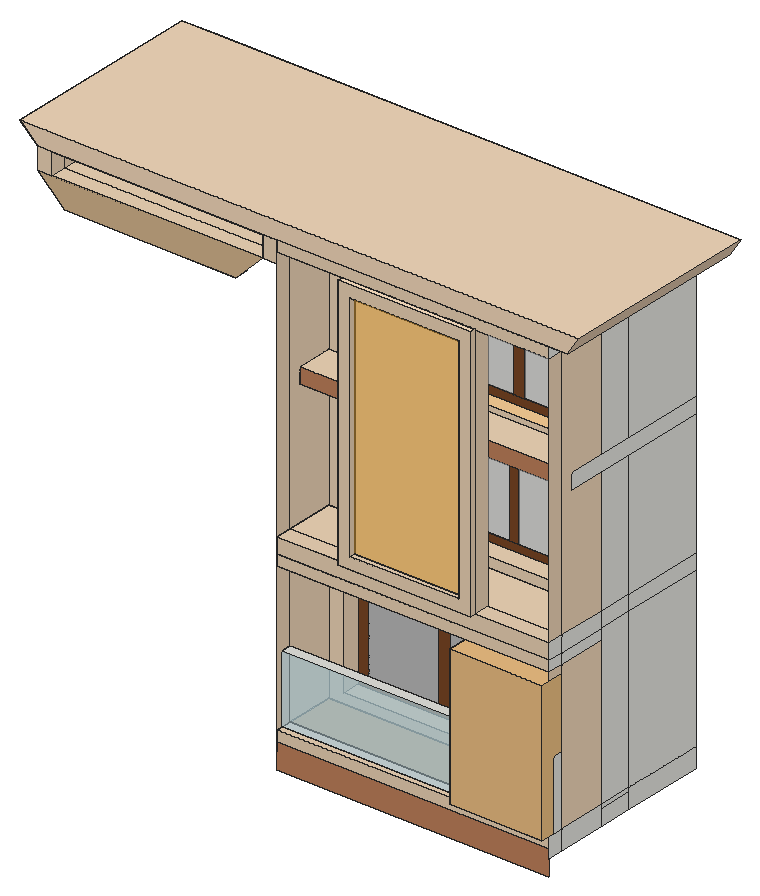
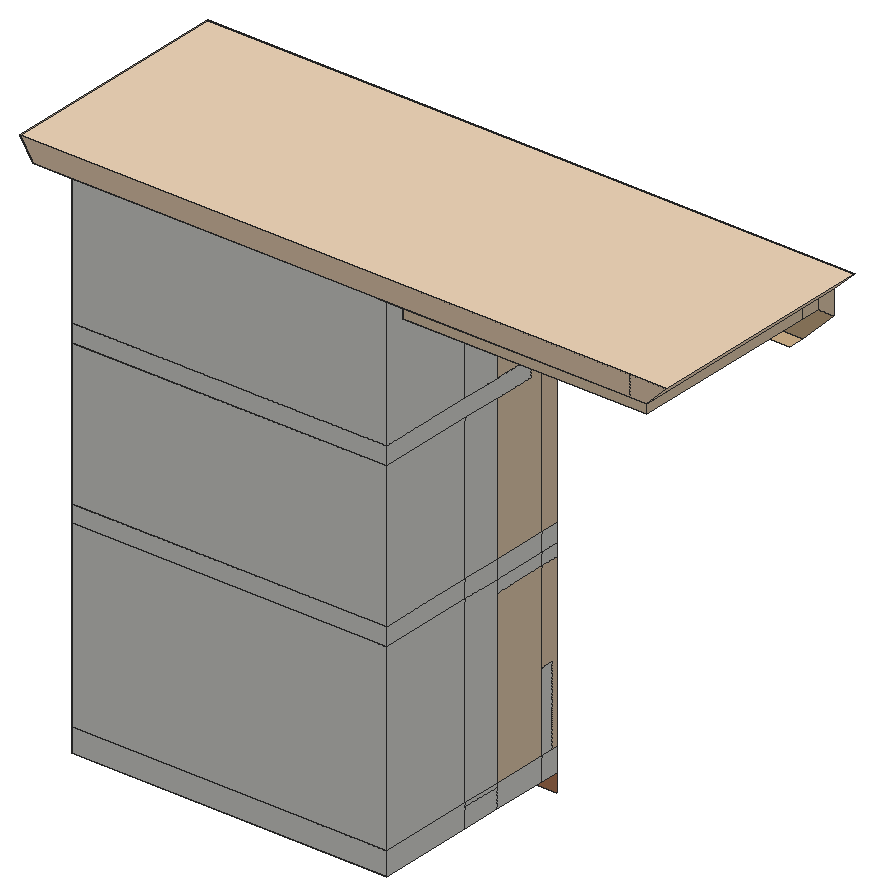
# SketchUp Ruby script. Lengths in inches.
U = 1.inch
M = Sketchup.active_model
def pt(a) = Geom::Point3d.new(a.map { |v| v * U })
def face(e, loops, mat)
  f = e.add_face(loops[0].map { |a| pt(a) })
  loops[1..].each { |l| e.add_face(l.map { |a| pt(a) }).erase! }
  f.material = f.back_material = mat if mat
  f
end
# faces: each face lists its corners as indices into pts; further lists are holes
def faces(e, pts, list, mat = nil) = list.each { |f| face(e, (f[0].is_a?(Array) ? f : [f]).map { |l| l.map { |i| pts[i] } }, mat) }
# xy, xz, yz: faces in a plane at the given z, y or x. An outline is a flat list of corners, or four numbers for a rectangle; further outlines are holes
def ring(l) = l.size == 4 ? [[l[0], l[1]], [l[2], l[1]], [l[2], l[3]], [l[0], l[3]]] : l.each_slice(2).to_a
def flat(e, list, mat, &to3) = list.each { |f| face(e, (f[0].is_a?(Array) ? f : [f]).map { |l| ring(l).map { |u, v| to3.(u, v) } }, mat) }
def xy(e, z, list, mat = nil) = flat(e, list, mat) { |x, y| [x, y, z] }
def xz(e, y, list, mat = nil) = flat(e, list, mat) { |x, z| [x, y, z] }
def yz(e, x, list, mat = nil) = flat(e, list, mat) { |y, z| [x, y, z] }
def lines(e, pts, list) = list.each { |a, b| e.add_line(pt(pts[a]), pt(pts[b])) }
# prism: a flat outline (further loops are holes) pulled along v
def prism(e, loops, v, mat = nil)
  f = face(e, loops, mat); d = Geom::Vector3d.new(v.map { |x| x * U })
  f.pushpull(f.normal.samedirection?(d) ? d.length : -d.length)
end
def box(e, o, s, mat = nil) = prism(e, [[o, [o[0] + s[0], o[1], o[2]], [o[0] + s[0], o[1] + s[1], o[2]], [o[0], o[1] + s[1], o[2]]]], [0, 0, s[2]], mat)
def at(x, y, z, deg = 0) = Geom::Transformation.translation(pt([x, y, z])) * Geom::Transformation.rotation(ORIGIN, Z_AXIS, deg.degrees)
def axes(o, x, y, z) = Geom::Transformation.new([*x, 0, *y, 0, *z, 0, *pt(o).to_a, 1])
def part(name) = M.definitions.add(name)
# library, detail: a bought-in or finely detailed component or shape, given as its bounding box
def library(name, o, s) = part(name).tap { |d| box(d.entities, o, s) }
def detail(e, o, s) = box(e.add_group.entities, o, s)
def put(e, d, t, mat = nil) = e.add_instance(d, t).tap { |i| i.material = mat if mat }
def group(e, t, mat = nil) = e.add_group.tap { |g| g.transformation = t; g.material = mat if mat }.entities
root = M.entities
M.materials.add("[0012_Bisque]").color = [234, 209, 180]
M.materials.add("[0012_Bisque]1").color = [237, 212, 182]
M.materials.add("[0012_Bisque]2").color = [242, 216, 186]
M.materials.add("[0012_Bisque]3").color = [255, 228, 196]
M.materials.add("[0035_Tan]").color = [210, 180, 140]
M.materials.add("[0036_BurlyWood]").color = [249, 207, 151]
M.materials.add("[0036_BurlyWood]1").color = [201, 166, 122]
M.materials.add("[Mirror 01]").color = [185, 185, 185]
M.materials.add("[Translucent Glass Gray]").color = [214, 214, 214]
M.materials["[Translucent Glass Gray]"].alpha = 0.5
M.materials.add("[Translucent Glass Safety]").color = [255, 178, 52]
M.materials["[Translucent Glass Safety]"].alpha = 0.5
M.materials.add("[Translucent Glass Safety]1").color = [204, 235, 244]
M.materials["[Translucent Glass Safety]1"].alpha = 0.5
M.materials.add("[Wood Veneer 01]").color = [120, 70, 37]
M.materials.add("[Wood Veneer 02]1").color = [190, 128, 91]
c1 = library("chau cay",[-24.34,-109.24,0],[56.46,62.58,79.69])
xy(root,211.6875,[[211.5,403.76,376.86,424.53],[211.5,424.53,376.86,475.86]])
xy(root,221.625,[[211.5,403.76,376.86,424.53]])
xy(root,223.75,[[211.5,367.9,376.86,374.19],[211.5,403.76,376.86,424.53],[211.5,424.53,376.86,475.86]])
xy(root,223.75,[[211.5,364.57,376.86,367.9]],"[0012_Bisque]")
xy(root,223.75,[[211.5,374.19,376.86,403.76]],"[0036_BurlyWood]1")
xy(root,229.55,[[220.36,403.76,373.55,414.89]],"[0012_Bisque]1")
xy(root,265.3125,[[211.5,367.9,376.86,374.19]])
xy(root,310.05,[[220.36,403.76,373.55,414.89]],"[0012_Bisque]1")
xy(root,313.0625,[[211.5,364.57,376.86,403.76]],"[0012_Bisque]")
xy(root,319.6875,[[211.5,364.57,376.86,403.76],[211.5,403.76,376.86,424.53],[211.5,424.53,376.86,475.86]])
xy(root,329,[[251.21,364.57,331.62,374.19],[211.5,403.76,376.86,424.53],[211.5,424.53,376.86,475.86]])
xy(root,329,[[211.5,364.57,251.21,374.19],[331.62,364.57,376.86,374.19]],"[0012_Bisque]")
xy(root,329,[[211.5,374.19,376.86,403.76]],"[0012_Bisque]1")
xy(root,329,[[251.21,361.2,331.62,364.57]],"[0012_Bisque]3")
xy(root,334.92,[[224.99,403.76,366.68,415.39]],"[0012_Bisque]1")
xy(root,335.97,[[258.17,361.2,324.65,364.57]],"[0012_Bisque]")
xy(root,394.98,[[224.99,403.76,366.68,415.39]],"[0012_Bisque]1")
xy(root,404.8125,[[211.5,403.76,376.86,424.53],[211.5,424.53,376.86,475.86]])
xy(root,404.8125,[[211.5,381.51,376.86,403.76]],"[0012_Bisque]1")
xy(root,414.0625,[[211.5,403.76,376.86,424.53],[211.5,424.53,376.86,475.86]])
xy(root,414.0625,[[211.5,381.51,376.86,403.76]],"[0012_Bisque]1")
xy(root,417.26,[[220.24,403.76,369.49,412.64]],"[0036_BurlyWood]")
xy(root,461.22,[[82.19,364.57,186.51,373.01]],"[0035_Tan]")
xy(root,476.97,[[258.17,361.2,324.65,364.57]],"[0012_Bisque]")
xy(root,477.4375,[[74.5,364.57,202.72,374.1875],[74.5,374.1875,202.72,476.36]],"[0012_Bisque]1")
xy(root,478.89,[[220.24,403.76,369.49,412.64]],"[0012_Bisque]1")
xy(root,483.9375,[[211.5,403.76,376.86,424.53],[211.5,424.53,376.86,475.86]])
xy(root,483.9375,[[211.5,364.57,211.5,403.76,376.86,403.76,376.86,364.57,331.62,364.57,331.62,374.19,251.21,374.19,251.21,364.57]],"[0012_Bisque]")
xy(root,483.9375,[[251.21,361.2,331.62,364.57]],"[0012_Bisque]3")
xy(root,490.375,[[65.97,364.57,74.5,487.49],[202.72,364.57,211.5,487.49],[211.5,364.57,376.86,475.86],[376.86,364.57,388.14,487.49],[211.5,475.86,376.86,487.49],
  [74.5,476.36,202.72,487.49]])
xy(root,490.375,[[74.5,364.57,202.72,476.36]],"[0012_Bisque]3")
xy(root,501.125,[[55.1,364.57,394.89,487.49]],"[0012_Bisque]2")
xz(root,361.2,[[[251.21,329,331.62,483.9375],[258.17,335.97,324.65,476.97]]],"[0012_Bisque]")
xz(root,364.57,[[[251.21,329,331.62,483.9375],[258.17,335.97,324.65,476.97]]])
xz(root,364.57,[[211.5,217.14,376.86,223.75],[211.5,313.0625,376.86,319.6875],[211.5,319.6875,376.86,329],[202.72,477.4375,211.5,490.375],[211.5,483.9375,376.86,490.375]],"[0012_Bisque]")
xz(root,364.57,[[65.97,477.4375,74.5,490.375]],"[0012_Bisque]1")
xz(root,364.57,[[65.97,490.375,388.14,490.375,394.89,501.125,55.1,501.125]],"[0012_Bisque]2")
xz(root,364.57,[[82.19,461.22,186.51,461.22,202.72,477.4375,65.97,477.4375]],"[0035_Tan]")
xz(root,364.57,[[258.17,335.97,324.65,476.97]],"[Translucent Glass Safety]")
xz(root,364.57,[[211.5,201.93,376.86,217.14]],"[Wood Veneer 02]1")
xz(root,367.9,[[211.5,223.75,376.86,265.3125]],"[Translucent Glass Safety]1")
xz(root,374.19,[[251.21,329,331.62,483.9375]],"[0012_Bisque]3")
xz(root,374.19,[[211.5,223.75,376.86,265.3125]],"[Translucent Glass Safety]1")
xz(root,381.51,[[211.5,404.8125,376.86,414.0625]],"[Wood Veneer 02]1")
xz(root,403.76,[[211.5,211.6875,376.86,221.625],[211.5,221.625,376.86,223.75],[211.5,313.0625,376.86,319.6875],[211.5,319.6875,376.86,329]])
xz(root,403.76,[[[211.5,223.75,376.86,313.0625],[220.36,229.55,373.55,310.05]],[[211.5,329,376.86,404.8125],[224.99,334.92,366.68,394.98]],[[211.5,414.0625,376.86,483.9375],[220.24,417.26,369.49,478.89]]],"[0012_Bisque]1")
xz(root,412.64,[[224.95,421.98,266.57,474.17],[273.5,421.98,316.82,474.17],[323.75,421.98,364.77,474.17]],"[Translucent Glass Gray]")
xz(root,412.64,[[[220.24,417.26,369.49,478.89],[224.95,421.98,364.77,474.17]],[266.57,421.98,273.5,474.17],[316.82,421.98,323.75,474.17]],"[Wood Veneer 01]")
xz(root,414.89,[[226.87,236.0625,268.98,303.54],[275.89,236.0625,318.42,303.54],[325.32,236.0625,367.04,303.54]],"[Mirror 01]")
xz(root,414.89,[[[220.36,229.55,373.55,310.05],[226.87,236.0625,367.04,303.54]],[268.98,236.0625,275.89,303.54],[318.42,236.0625,325.32,303.54]],"[Wood Veneer 01]")
xz(root,415.39,[[229.47,339.4,267.77,390.5],[273.57,339.4,312.08,390.5],[317.88,339.4,362.2,390.5]],"[Translucent Glass Gray]")
xz(root,415.39,[[[224.99,334.92,366.68,394.98],[229.47,339.4,362.2,390.5]],[267.77,339.4,273.57,390.5],[312.08,339.4,317.88,390.5]],"[Wood Veneer 01]")
xz(root,424.53,[[211.5,211.6875,376.86,221.625],[211.5,221.625,376.86,223.75],[211.5,223.75,376.86,319.6875],[211.5,319.6875,376.86,329],[211.5,329,376.86,404.8125],
  [211.5,414.0625,376.86,483.9375]])
xz(root,475.86,[[211.5,211.6875,376.86,223.75],[211.5,223.75,376.86,319.6875],[211.5,319.6875,376.86,329],[211.5,329,376.86,404.8125],[211.5,404.8125,376.86,414.0625],
  [211.5,414.0625,376.86,483.9375],[211.5,483.9375,376.86,490.375]])
xz(root,476.36,[[74.5,477.4375,202.72,490.375]],"[0012_Bisque]1")
xz(root,487.49,[[65.97,490.375,55.1,501.125,74.5,501.125,74.5,490.375],[74.5,490.375,74.5,501.125,394.89,501.125,388.14,490.375]],"[0012_Bisque]2")
yz(root,74.5,[[364.57,477.4375,374.1875,490.375],[374.1875,477.4375,476.36,490.375]],"[0012_Bisque]1")
yz(root,202.72,[[364.57,477.4375,374.1875,490.375],[374.1875,477.4375,476.36,490.375]],"[0012_Bisque]1")
yz(root,211.5,[[364.57,211.6875,374.19,223.75],[374.19,211.6875,403.76,223.75],[403.76,211.6875,424.53,221.625],[424.53,211.6875,475.86,223.75],[403.76,221.625,424.53,223.75],
  [367.9,223.75,374.19,265.3125],[403.76,223.75,424.53,319.6875],[424.53,223.75,475.86,319.6875],[364.57,313.0625,374.19,319.6875],[374.19,313.0625,403.76,319.6875],
  [364.57,319.6875,374.19,329],[374.19,319.6875,403.76,329],[403.76,319.6875,424.53,329],[424.53,319.6875,475.86,329],[403.76,329,424.53,404.8125],
  [424.53,329,475.86,404.8125],[381.51,404.8125,475.86,414.0625],[403.76,414.0625,424.53,483.9375],[424.53,414.0625,475.86,483.9375],[364.57,483.9375,374.19,490.375],
  [374.19,483.9375,403.76,490.375],[403.76,483.9375,424.53,490.375],[424.53,483.9375,475.86,490.375]])
yz(root,211.5,[[364.57,223.75,367.9,223.75,367.9,265.3125,374.19,265.3125,374.19,313.0625,364.57,313.0625],[364.57,329,374.19,483.9375]],"[0012_Bisque]")
yz(root,211.5,[[374.19,223.75,403.76,313.0625],[374.19,329,403.76,329,403.76,404.8125,381.51,404.8125,381.51,414.0625,403.76,414.0625,403.76,483.9375,374.19,483.9375]],"[0012_Bisque]1")
yz(root,220.24,[[403.76,417.26,412.64,478.89]],"[0036_BurlyWood]")
yz(root,220.36,[[403.76,229.55,414.89,310.05]],"[0012_Bisque]1")
yz(root,224.99,[[403.76,334.92,415.39,394.98]],"[0012_Bisque]1")
yz(root,251.21,[[361.2,329,364.57,483.9375],[364.57,329,374.19,483.9375]],"[0012_Bisque]")
yz(root,258.17,[[361.2,335.97,364.57,476.97]],"[0012_Bisque]")
yz(root,324.65,[[361.2,335.97,364.57,476.97]],"[0012_Bisque]")
yz(root,331.62,[[361.2,329,364.57,483.9375],[364.57,329,374.19,483.9375]],"[0012_Bisque]")
yz(root,366.68,[[403.76,334.92,415.39,394.98]],"[0012_Bisque]1")
yz(root,369.49,[[403.76,417.26,412.64,478.89]],"[0012_Bisque]1")
yz(root,373.55,[[403.76,229.55,414.89,310.05]],"[0012_Bisque]1")
yz(root,376.86,[[364.57,211.6875,374.19,223.75],[374.19,211.6875,403.76,223.75],[403.76,211.6875,424.53,221.625],[424.53,211.6875,475.86,223.75],[403.76,221.625,424.53,223.75],
  [367.9,223.75,374.19,265.3125],[403.76,223.75,424.53,319.6875],[424.53,223.75,475.86,319.6875],[364.57,313.0625,374.19,319.6875],[374.19,313.0625,403.76,319.6875],
  [364.57,319.6875,374.19,329],[374.19,319.6875,403.76,329],[403.76,319.6875,424.53,329],[424.53,319.6875,475.86,329],[403.76,329,424.53,404.8125],
  [424.53,329,475.86,404.8125],[381.51,404.8125,475.86,414.0625],[403.76,414.0625,424.53,483.9375],[424.53,414.0625,475.86,483.9375],[364.57,483.9375,374.19,490.375],
  [374.19,483.9375,403.76,490.375],[403.76,483.9375,424.53,490.375],[424.53,483.9375,475.86,490.375]])
yz(root,376.86,[[364.57,223.75,364.57,313.0625,374.19,313.0625,374.19,265.3125,367.9,265.3125,367.9,223.75],[364.57,329,374.19,483.9375]],"[0012_Bisque]")
yz(root,376.86,[[374.19,223.75,403.76,313.0625],[374.19,329,374.19,483.9375,403.76,483.9375,403.76,414.0625,381.51,414.0625,381.51,404.8125,403.76,404.8125,403.76,329]],"[0012_Bisque]1")
p = [[65.97,364.57,490.375],[55.1,364.57,501.125],[55.1,487.49,501.125],[65.97,487.49,490.375],[394.89,364.57,501.125],[388.14,364.57,490.375],
  [388.14,487.49,490.375],[394.89,487.49,501.125]]
faces(root,p,[[0,1,2,3],[4,5,6,7]],"[0012_Bisque]2")
put(root,c1,axes([344.74,468.5,223.75],[1,0,0],[0,1,0],[0,0,1.06]))
